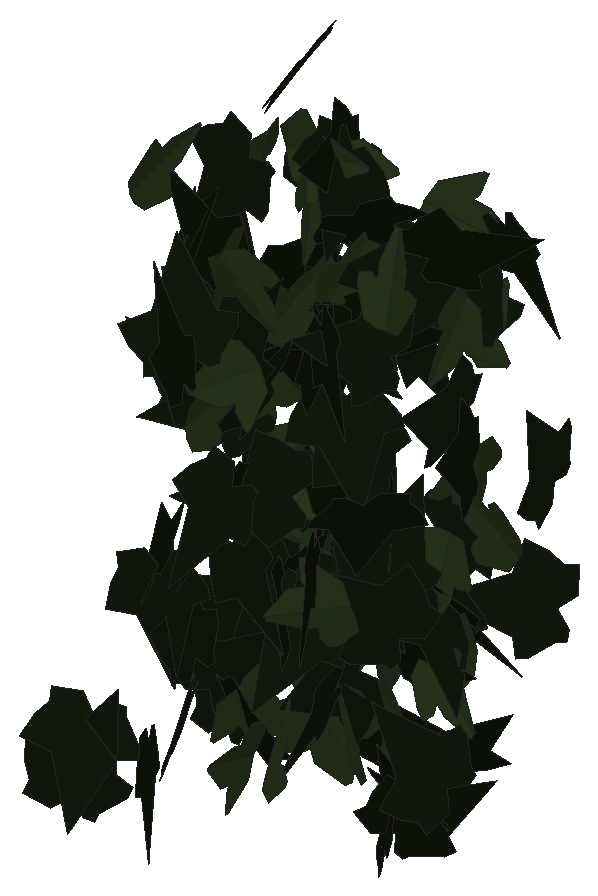
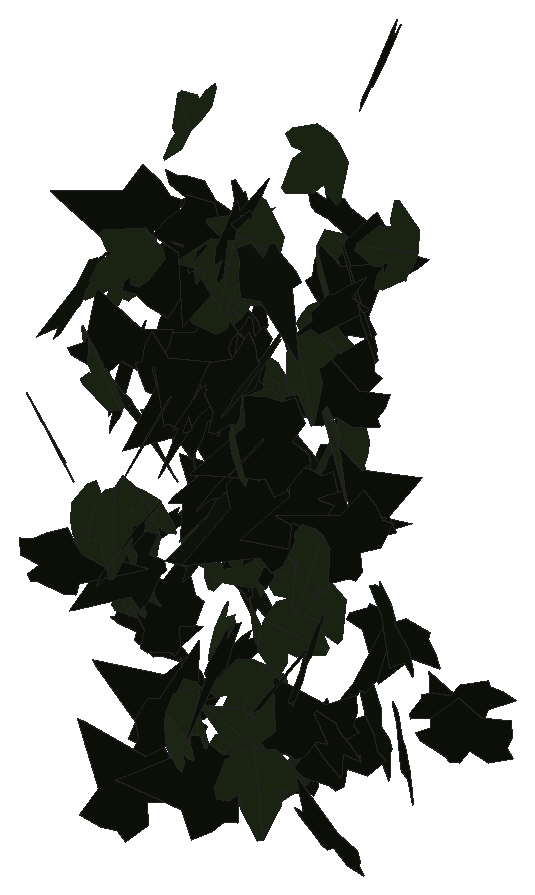
# SketchUp Ruby script. Lengths in inches.
U = 1.inch
M = Sketchup.active_model
def pt(a) = Geom::Point3d.new(a.map { |v| v * U })
def face(e, loops, mat)
  f = e.add_face(loops[0].map { |a| pt(a) })
  loops[1..].each { |l| e.add_face(l.map { |a| pt(a) }).erase! }
  f.material = f.back_material = mat if mat
  f
end
# faces: each face lists its corners as indices into pts; further lists are holes
def faces(e, pts, list, mat = nil) = list.each { |f| face(e, (f[0].is_a?(Array) ? f : [f]).map { |l| l.map { |i| pts[i] } }, mat) }
# xy, xz, yz: faces in a plane at the given z, y or x. An outline is a flat list of corners, or four numbers for a rectangle; further outlines are holes
def ring(l) = l.size == 4 ? [[l[0], l[1]], [l[2], l[1]], [l[2], l[3]], [l[0], l[3]]] : l.each_slice(2).to_a
def flat(e, list, mat, &to3) = list.each { |f| face(e, (f[0].is_a?(Array) ? f : [f]).map { |l| ring(l).map { |u, v| to3.(u, v) } }, mat) }
def xy(e, z, list, mat = nil) = flat(e, list, mat) { |x, y| [x, y, z] }
def xz(e, y, list, mat = nil) = flat(e, list, mat) { |x, z| [x, y, z] }
def yz(e, x, list, mat = nil) = flat(e, list, mat) { |y, z| [x, y, z] }
def lines(e, pts, list) = list.each { |a, b| e.add_line(pt(pts[a]), pt(pts[b])) }
# prism: a flat outline (further loops are holes) pulled along v
def prism(e, loops, v, mat = nil)
  f = face(e, loops, mat); d = Geom::Vector3d.new(v.map { |x| x * U })
  f.pushpull(f.normal.samedirection?(d) ? d.length : -d.length)
end
def box(e, o, s, mat = nil) = prism(e, [[o, [o[0] + s[0], o[1], o[2]], [o[0] + s[0], o[1] + s[1], o[2]], [o[0], o[1] + s[1], o[2]]]], [0, 0, s[2]], mat)
def at(x, y, z, deg = 0) = Geom::Transformation.translation(pt([x, y, z])) * Geom::Transformation.rotation(ORIGIN, Z_AXIS, deg.degrees)
def axes(o, x, y, z) = Geom::Transformation.new([*x, 0, *y, 0, *z, 0, *pt(o).to_a, 1])
def part(name) = M.definitions.add(name)
# library, detail: a bought-in or finely detailed component or shape, given as its bounding box
def library(name, o, s) = part(name).tap { |d| box(d.entities, o, s) }
def detail(e, o, s) = box(e.add_group.entities, o, s)
def put(e, d, t, mat = nil) = e.add_instance(d, t).tap { |i| i.material = mat if mat }
def group(e, t, mat = nil) = e.add_group.tap { |g| g.transformation = t; g.material = mat if mat }.entities
root = M.entities
M.materials.add("efeu1").color = [18, 25, 13]
M.materials.add("efeu2").color = [43, 57, 29]
c1 = part("ivyleaf_10")
p = [[0,0.5,-0.03],[-0.0625,2.02,-0.43],[-0.19,2.01,-0.46],[-0.54,1.05,-0.29],[-0.52,0.625,-0.18],[-0.83,0.76,-0.28],
  [-1.16,0.64,-0.33],[-1.15,0.33,-0.24],[-0.77,-0.39,0.02],[-0.3,-0.51,0.16],[0.04,-0.48,0.23],[-0.02,2.01,-0.4375],
  [-0.06,2.01,-0.43],[0.04,-0.49,0.23],[0.67,-0.49,0.14],[1.38,0.36,-0.2],[1.375,0.51,-0.24],[0.81,0.65,-0.19],
  [0.62,0.59,-0.15],[0.6,1.09,-0.28],[0.5,1.23,-0.31]]
faces(c1.entities,p,[[0,1,2,3,4,5,6,7,8,9,10],[11,12,0,13,14,15,16,17,18,19,20]],"efeu2")
c2 = part("ivyleaf_9")
p = [[1.54,2.16,1.25],[1.36,2.04,1.19],[-0.21,0.99,0.68],[-0.71,1.11,0.82],[-0.85,0.86,0.67],[-0.8,0.17,0.21],
  [-0.9,-0.01,0.1],[-0.67,-0.16,-0.02],[-0.08,-0.08,-0.05],[-0.03,-0.6,-0.4],[0.65,-0.88,-0.66],[0.83,-0.6,-0.49],
  [1.29,-0.42,-0.43],[1.8125,-0.07,-0.26],[1.21,0.44,0.15]]
faces(c2.entities,p,[[0,1,2,3,4,5,6,7,8,9,10,11,12,13,14]],"efeu1")
put(root,c1,axes([39.3,222.3,218.73],[-0.44801,0.21551,-0.05329],[0.04622,-0.02685,-0.49713],[-0.21713,-0.45037,0.00414]))
put(root,c2,axes([39.62,220.08,216.47],[-0.0302,0.25565,0.42864],[-0.09039,0.41952,-0.25658],[-0.49083,-0.09298,0.02087]))
put(root,c2,axes([39.49,221.64,213.66],[-0.36439,0.2665,0.21494],[0.16582,-0.13726,0.45129],[0.29954,0.40017,0.01165]))
put(root,c2,axes([39.87,220.75,218.66],[0.00532,0.02765,0.49921],[-0.44859,0.22071,-0.00744],[-0.22077,-0.4478,0.02716]))
put(root,c2,axes([39.52,218.93,214.83],[-0.25585,-0.4171,-0.10278],[0.05191,0.08873,-0.48932],[0.42643,-0.26106,-0.0021]))
put(root,c2,axes([39.48,218.61,213.9],[-0.34655,0.01099,0.36026],[0.35709,-0.05735,0.34525],[0.04891,0.49658,0.0319]))
put(root,c2,axes([39.36,221.26,218.25],[-0.01472,-0.00947,0.49969],[0.43968,0.23744,0.01745],[-0.23762,0.43992,0.00133]))
put(root,c2,axes([39.3125,222.43,217],[0.20074,-0.12423,-0.44076],[0.38837,-0.20881,0.23573],[-0.24265,-0.43699,0.01266]))
put(root,c1,axes([39.67,222.1,221.64],[0.0543,-0.49697,-0.00844],[0.00005,0.0085,-0.49993],[0.49704,0.05429,0.00097]))
put(root,c1,axes([39.84,221.24,220.02],[0.29275,-0.37958,-0.14219],[-0.0842,0.11462,-0.47934],[0.39649,0.3046,0.00319]))
put(root,c2,axes([40.08,221.4375,218.42],[-0.2695,-0.1346,0.39906],[-0.36868,-0.15361,-0.30079],[0.20357,-0.45639,-0.01645]))
put(root,c2,axes([39.66,220.1,216.45],[-0.28436,-0.21441,-0.35096],[0.28393,0.20633,-0.3561],[0.29753,-0.40181,0.00441]))
put(root,c1,axes([39.79,219.7,222.21],[0.08797,-0.2433,0.42786],[-0.05521,0.42702,0.25418],[-0.48909,-0.09197,0.04826]))
put(root,c1,axes([39.93,222.3,217.27],[-0.07929,-0.27273,0.4115],[-0.01679,-0.41504,-0.27831],[0.49339,-0.05795,0.05666]))
put(root,c2,axes([39.73,221.55,218.81],[0.16954,0.19203,0.42939],[0.26115,0.3412,-0.2557],[-0.39122,0.31098,0.0154]))
put(root,c2,axes([39.91,221.53,215.5],[-0.41786,-0.09545,-0.25745],[0.25174,0.05399,-0.42862],[0.10962,-0.48783,0.00293]))
put(root,c2,axes([40.07,220.25,215.38],[-0.12429,-0.3751,0.30635],[0.08668,0.29395,0.39507],[-0.47648,0.15132,-0.00804]))
put(root,c2,axes([39.74,222.57,216.5625],[0.14211,-0.47646,0.05281],[0.01344,-0.0511,-0.4972],[0.47919,0.14273,-0.00172]))
put(root,c2,axes([39.97,221.43,221.81],[-0.14993,-0.39085,0.27341],[-0.1041,-0.25288,-0.41859],[0.46549,-0.18244,-0.00554]))
put(root,c2,axes([39.9375,221.49,215.15],[-0.27909,-0.10822,0.4005],[0.37157,0.14948,0.29932],[-0.18452,0.4647,-0.00302]))
put(root,c2,axes([40.23,222.23,222.99],[-0.21232,0.44741,-0.06886],[0.02994,-0.06201,-0.49524],[-0.45169,-0.21442,-0.00046]))
put(root,c2,axes([40.08,220.82,220],[-0.41487,-0.07019,0.2701],[0.27115,0.01306,0.41989],[-0.066,0.49488,0.02723]))
put(root,c1,axes([40.17,221.32,218.69],[-0.35539,-0.35047,-0.02948],[0.02232,0.01935,-0.49913],[0.351,-0.35609,0.00189]))
put(root,c2,axes([40.27,219.6,214.38],[0.0029,0.19478,0.46049],[-0.01837,0.46023,-0.19455],[-0.49965,-0.01579,0.00983]))
put(root,c2,axes([39.84,220.9375,214.51],[-0.12861,0.01441,0.48296],[0.46818,-0.11982,0.12825],[0.11943,0.48522,0.01733]))
put(root,c2,axes([39.93,219.54,214.26],[-0.1694,0.00721,-0.47038],[0.46317,-0.08493,-0.1681],[-0.08232,-0.49268,0.02209]))
put(root,c2,axes([39.96,220.1875,220.98],[-0.07585,0.32165,0.37522],[0.08774,-0.36482,0.33047],[0.48636,0.11598,-0.0011]))
put(root,c1,axes([40.1,221.24,217.28],[-0.36769,-0.11561,-0.31849],[0.30097,0.10443,-0.38537],[0.15563,-0.47511,-0.0072]))
put(root,c1,axes([40.41,222.23,214.8125],[-0.41323,-0.27054,0.07777],[-0.06222,-0.04694,-0.49389],[0.27454,-0.41785,0.00513]))
put(root,c2,axes([40.0625,221.9375,220.04],[0.29327,0.19818,0.35315],[0.29639,0.19208,-0.35392],[-0.27595,0.41693,-0.00481]))
put(root,c2,axes([40.24,221.3,219.01],[0.33732,0.35149,0.11258],[0.07116,0.08772,-0.48708],[-0.36215,0.34462,0.00916]))
put(root,c2,axes([40.08,222.17,218.9375],[0.43106,0.14291,0.20921],[0.19332,0.08134,-0.45388],[-0.16376,0.47219,0.01487]))
put(root,c1,axes([40.43,219.97,218.95],[0.07725,-0.04196,0.49221],[-0.15093,0.47237,0.06396],[-0.47037,-0.15846,0.06032]))
put(root,c2,axes([40.67,220.06,221.18],[0.12898,-0.07058,0.47789],[-0.36175,0.31371,0.14396],[-0.32016,-0.38289,0.02986]))
put(root,c2,axes([40.17,222.55,221.35],[0.17411,-0.45097,0.12772],[0.04085,-0.12113,-0.48338],[0.46692,0.17875,-0.00534]))
put(root,c1,axes([40.49,220.76,214.69],[-0.14852,-0.36538,-0.30731],[0.13502,0.27656,-0.39406],[0.45794,-0.20004,0.01652]))
put(root,c2,axes([40.82,220.82,219.2],[-0.3644,0.34211,-0.01318],[0.00909,-0.00958,-0.49983],[-0.34224,-0.36452,0.00076]))
put(root,c1,axes([40.55,222.375,220.14],[0.17648,-0.40184,0.23955],[0.08987,-0.22214,-0.43884],[0.45911,0.19794,-0.00618]))
put(root,c2,axes([40.95,221.02,217.57],[-0.25824,-0.07879,0.42084],[-0.39445,-0.14735,-0.26963],[0.16651,-0.47125,0.01395]))
put(root,c2,axes([40.5,222.59,219.71],[0.10549,-0.48701,0.04114],[0.0131,-0.03925,-0.49828],[0.48857,0.1062,0.00448]))
put(root,c1,axes([40.67,221.24,219.85],[0.01529,-0.32853,0.37661],[-0.0147,0.37632,0.32888],[-0.49955,-0.02113,0.00185]))
put(root,c2,axes([40.41,220.83,214.29],[0.14982,-0.18464,0.43985],[0.27098,-0.34648,-0.23774],[0.39258,0.30962,-0.00375]))
put(root,c2,axes([40.73,219.92,219.69],[-0.12789,-0.13533,0.46404],[0.41546,0.21457,0.17707],[-0.24706,0.43087,0.05757]))
put(root,c2,axes([40.61,222.33,220.78],[0.22982,-0.28587,0.3398],[0.22344,-0.2562,-0.36666],[0.38374,0.32038,0.00999]))
put(root,c2,axes([40.97,222.2,216.6],[0.23182,-0.19665,-0.39697],[-0.3012,0.25858,-0.30399],[0.32486,0.38008,0.00142]))
put(root,c1,axes([40.89,221.42,217.42],[0.42368,0.16613,-0.20712],[0.13566,0.19983,0.43779],[0.22824,-0.42716,0.12425]))
put(root,c1,axes([40.78,221.6,214.71],[-0.23927,-0.13519,0.4177],[0.36256,0.20744,0.27481],[-0.2476,0.43439,-0.00124]))
put(root,c1,axes([41.05,219.85,221.7],[0.20607,-0.42795,0.15619],[0.07588,-0.13679,-0.4749],[0.4492,0.21943,0.00856]))
put(root,c2,axes([41.1875,219.48,218.49],[-0.17767,0.21448,-0.41525],[0.27559,-0.31071,-0.2784],[-0.37747,-0.3278,-0.00781]))
put(root,c2,axes([41.38,218.5,220.91],[-0.46383,-0.1176,0.14502],[0.14023,0.03697,0.47851],[-0.12327,0.48457,-0.00131]))
put(root,c1,axes([41.03,221.45,216.75],[0.32857,-0.20091,0.31887],[0.27158,-0.1671,-0.38513],[0.26131,0.42628,-0.00068]))
put(root,c1,axes([41.57,219.36,220.27],[0.29202,-0.0677,-0.40017],[-0.38726,0.10107,-0.2997],[0.12147,0.48498,0.0066]))
put(root,c1,axes([41.26,221.2,222.07],[-0.02616,0.43415,-0.24663],[0.00712,-0.24662,-0.43489],[-0.49926,-0.02626,0.00672]))
put(root,c1,axes([41.43,221.29,214.36],[-0.33069,-0.36139,-0.1002],[0.068,0.0736,-0.48986],[0.36881,-0.33761,0.00047]))
put(root,c1,axes([41.07,221.15,222.43],[-0.08189,-0.04115,0.49153],[0.4757,0.12512,0.08973],[-0.13038,0.48234,0.01866]))
put(root,c2,axes([41.18,221.34,217.28],[-0.05181,0.06609,0.4929],[0.30622,-0.38623,0.08398],[0.39185,0.31057,-0.00046]))
put(root,c2,axes([41.45,222.0625,220.375],[0.24263,-0.31489,-0.30327],[-0.18063,0.24365,-0.3975],[0.39812,0.30245,0.00448]))
put(root,c2,axes([41.54,221.49,222.3125],[-0.01556,-0.08629,0.49225],[-0.14127,-0.47164,-0.08715],[0.47938,-0.14179,-0.00971]))
put(root,c1,axes([41.52,221.37,222.33],[0.31445,0.38338,0.06432],[0.04083,0.0497,-0.49585],[-0.38659,0.31709,-0.00005]))
put(root,c2,axes([41.33,221.94,214.16],[0.15993,0.15414,-0.44796],[0.28679,0.34481,0.22103],[0.37706,-0.32764,0.02188]))
put(root,c1,axes([41.6875,220.61,215.0625],[-0.35445,-0.27769,-0.21739],[0.16749,0.13868,-0.45024],[0.31034,-0.39199,-0.00529]))
put(root,c2,axes([41.66,221.41,222.51],[-0.08244,-0.48339,0.09766],[-0.02195,-0.09533,-0.49034],[0.49267,-0.08514,-0.0055]))
put(root,c2,axes([41.51,221.81,218.01],[0.31439,-0.38067,0.07904],[0.05027,-0.061,-0.49371],[0.38553,0.31838,-0.00009]))
put(root,c1,axes([41.78,222.27,215.09],[0.14468,-0.38115,0.28947],[0.09589,-0.27319,-0.40764],[0.46891,0.17347,-0.00595]))
put(root,c2,axes([41.92,220.4,220.33],[0.05014,-0.05989,-0.49386],[-0.35717,0.34118,-0.07763],[0.34629,0.36057,-0.00856]))
put(root,c2,axes([42.12,222.1875,220.19],[0.07208,-0.09724,0.48513],[-0.32056,0.36426,0.12065],[-0.37689,-0.32842,-0.00983]))
put(root,c2,axes([41.95,219.76,217.26],[-0.06999,0.13346,-0.47675],[-0.19823,0.43365,0.1505],[0.45366,0.21008,-0.00779]))
put(root,c1,axes([41.99,220.33,217.33],[0.1091,-0.4869,-0.03201],[-0.00697,0.03125,-0.49897],[0.4879,0.10932,0.00003]))
put(root,c2,axes([41.78,221.34,218.62],[0.05428,-0.42395,-0.25947],[-0.00199,0.26082,-0.42658],[0.49704,0.04734,0.02662]))
put(root,c2,axes([41.95,221.13,215.35],[0.13326,-0.29625,-0.3801],[0.1467,-0.35071,0.32478],[-0.45904,-0.19808,-0.00655]))
put(root,c1,axes([42.31,221.41,214.74],[0.02369,-0.01707,-0.49915],[-0.34222,0.36341,-0.02867],[0.36377,0.34299,0.00554]))
put(root,c2,axes([42.08,221.64,219.99],[-0.09063,0.17684,-0.45882],[-0.19573,0.41502,0.19862],[0.45108,0.21561,-0.006]))
put(root,c2,axes([41.65,220.87,220.19],[0.1538,-0.04409,-0.47371],[0.44104,0.19991,0.12458],[0.17842,-0.45617,0.10038]))
put(root,c2,axes([41.96,220.94,219.3],[-0.15577,-0.41624,-0.22908],[0.10804,0.20373,-0.44365],[0.46267,-0.18771,0.02647]))
put(root,c1,axes([42.03,220.78,221.04],[-0.04763,-0.45093,0.21069],[0.02318,0.20941,0.45344],[-0.49719,0.05296,0.00095]))
put(root,c1,axes([42.03,219.93,216.53],[0.29242,0.33978,-0.22144],[0.12995,0.18011,0.44796],[0.38419,-0.31954,0.01703]))
put(root,c2,axes([42.15,221.93,220.02],[0.30808,-0.29687,-0.25875],[-0.1782,0.18787,-0.42772],[0.35118,0.35577,0.00995]))
put(root,c2,axes([42.29,220.7,222.14],[0.28606,0.40883,-0.03206],[-0.0204,-0.02485,-0.49897],[-0.40958,0.28677,0.00247]))
put(root,c2,axes([41.92,221.09,220.17],[0.20062,-0.04302,0.45596],[0.45416,-0.04553,-0.20413],[0.05909,0.49606,0.02081]))
put(root,c1,axes([42,221.16,217.24],[0.09299,-0.11253,0.47821],[0.47523,-0.10276,-0.11659],[0.12453,0.47621,0.08785]))
put(root,c1,axes([42.2,218.42,222.375],[-0.39768,0.09056,-0.28923],[0.28393,-0.05558,-0.40779],[-0.10601,-0.48858,-0.00721]))
put(root,c2,axes([42.13,219.53,217.3],[0.13525,-0.09251,-0.47239],[0.42468,-0.20808,0.16234],[-0.22662,-0.44514,0.02229]))
put(root,c2,axes([42.33,220.3,217.45],[-0.00424,-0.28361,-0.41176],[0.08206,0.4058,-0.28035],[0.4932,-0.06995,0.0431]))
put(root,c2,axes([42.27,222.38,213.74],[0.38943,0.30413,-0.07651],[0.06025,0.04715,0.49411],[0.30776,-0.39406,0.00008]))
put(root,c2,axes([42.68,219.39,217.24],[-0.41022,-0.28537,-0.017],[0.01689,0.0055,-0.49968],[0.28537,-0.41053,0.00513]))
put(root,c1,axes([42.86,220.01,214.91],[-0.25583,0.298,-0.30943],[-0.2031,0.23345,0.39275],[0.37855,0.32664,0.0016]))
put(root,c2,axes([42.83,219.56,216.07],[-0.38792,0.20739,-0.23771],[0.19593,-0.13689,-0.43917],[-0.24724,-0.43388,0.02494]))
put(root,c2,axes([43.09,221.24,221.45],[-0.12697,-0.12506,-0.46716],[-0.27881,-0.37572,0.17636],[-0.39515,0.30528,0.02567]))
put(root,c2,axes([42.56,217.97,218.72],[0.2473,-0.39665,-0.17752],[-0.08825,0.15416,-0.46738],[0.4255,0.2625,0.00624]))
put(root,c1,axes([42.88,222.26,218.16],[-0.08173,-0.48524,-0.08866],[0.02918,0.08495,-0.49187],[0.49241,-0.08557,0.01443]))
put(root,c1,axes([42.82,217.89,215.86],[-0.04996,-0.15787,-0.47179],[-0.03187,-0.47217,0.16137],[-0.49648,0.04619,0.03712]))
put(root,c2,axes([42.76,219.66,216.99],[-0.16303,-0.09729,0.46256],[0.42096,0.19264,0.18888],[-0.21497,0.45103,0.0191]))
put(root,c2,axes([43.3,221.44,219.34],[-0.30657,0.33204,0.21393],[-0.13759,0.16407,-0.45183],[-0.37025,-0.3359,-0.00923]))
put(root,c2,axes([42.98,220.98,213.82],[0.40686,-0.24652,0.15392],[-0.13023,0.08208,0.47571],[-0.25981,-0.42719,0.00258]))
put(root,c2,axes([43.2,220.15,213.79],[0.00324,0.05013,0.49747],[-0.0734,0.49214,-0.04911],[-0.49457,-0.07271,0.01055]))
put(root,c2,axes([42.87,222.16,217.39],[-0.00839,-0.41309,0.28158],[-0.01014,-0.28142,-0.41316],[0.49983,-0.01265,-0.00365]))
put(root,c2,axes([43.16,216.15,222.18],[-0.03414,-0.36425,0.34082],[0.03003,0.3395,0.36584],[-0.49793,0.04545,-0.0013]))
put(root,c2,axes([43.03,221.9375,220.35],[-0.36778,-0.10519,0.32198],[0.31973,0.04911,0.38126],[-0.11183,0.48634,0.03115]))
put(root,c1,axes([42.875,221.6875,221.99],[0.09586,0.26838,0.41083],[0.13793,0.38698,-0.28499],[-0.47094,0.16797,0.00016]))
put(root,c2,axes([42.7,221.13,215.86],[0.1483,-0.12018,0.46213],[0.36603,-0.28214,-0.19083],[0.30664,0.39491,0.0043]))
put(root,c1,axes([42.91,222.35,220],[0.38893,-0.20551,-0.23769],[0.20985,-0.11163,0.43989],[-0.23387,-0.44193,-0.00058]))
put(root,c2,axes([43.45,219.93,218.49],[-0.01857,-0.00101,-0.49965],[-0.4824,0.1303,0.01766],[0.13018,0.48272,-0.00581]))
put(root,c2,axes([42.9375,219.23,221.37],[-0.09035,-0.02406,-0.49118],[0.49169,-0.01333,-0.08979],[-0.00877,-0.49924,0.02607]))
put(root,c1,axes([43.64,221.94,217.4375],[-0.25835,0.09063,-0.41838],[-0.39853,0.12751,0.27371],[0.15631,0.4749,0.00636]))
put(root,c2,axes([43.44,216.76,220.4],[-0.48223,-0.0677,-0.11345],[0.11221,0.01678,-0.48696],[0.06974,-0.49511,-0.00099]))
put(root,c1,axes([43.7,221.11,216.37],[0.09211,-0.09285,-0.48259],[-0.34654,0.33588,-0.13076],[0.34847,0.35856,-0.00247]))
put(root,c1,axes([43.36,221.08,217.59],[0.48804,-0.10562,0.02572],[0.02562,-0.00319,-0.49933],[0.10565,0.48871,0.0023]))
put(root,c2,axes([43.18,221.2,216.8125],[0.49333,-0.06311,0.05138],[0.05108,-0.00558,-0.49735],[0.06335,0.49597,0.00094]))
put(root,c2,axes([43.22,220.41,213.87],[0.00895,-0.04662,0.49774],[0.49893,0.0322,-0.00596],[-0.0315,0.49678,0.04709]))
put(root,c2,axes([43.95,219.25,221.39],[-0.33245,0.13964,0.34637],[-0.32486,0.12064,-0.36044],[-0.18424,-0.4647,0.01051]))
put(root,c2,axes([43.4,220.98,216.95],[0.04606,-0.48878,-0.0947],[-0.00884,0.09429,-0.49095],[0.4978,0.0469,0.00004]))
put(root,c2,axes([43.32,222.4375,221.53],[0.32348,-0.38054,-0.02339],[-0.0164,0.01676,-0.49945],[0.38091,0.32389,-0.00164]))
put(root,c1,axes([44,218.14,218.33],[-0.16148,-0.05636,0.46984],[-0.42357,-0.20412,-0.17006],[0.21098,-0.45294,0.01818]))
put(root,c2,axes([44.04,220.26,214.875],[-0.42559,-0.14105,-0.2213],[-0.20835,-0.07475,0.44833],[-0.15956,0.47383,0.00485]))
put(root,c1,axes([43.32,220.95,215.97],[0.24827,-0.00908,0.43391],[0.43365,-0.01512,-0.24843],[0.01763,0.49969,0.00036]))
put(root,c2,axes([43.66,219.53,217.97],[-0.36764,0.00764,0.33879],[0.33654,-0.05035,0.36634],[0.03971,0.4974,0.03188]))
put(root,c1,axes([43.69,221.07,221.08],[0.01424,0.30388,-0.39681],[-0.03519,-0.39537,-0.30404],[-0.49856,0.03659,0.01012]))
put(root,c2,axes([43.36,220.91,221.85],[0.15194,-0.01798,0.47602],[0.47635,0.00419,-0.15189],[0.00147,0.49966,0.0184]))
put(root,c2,axes([43.96,218.78,219.4375],[0.18677,0.40634,-0.22363],[-0.08875,-0.20531,-0.44718],[-0.45524,0.20673,-0.00457]))
put(root,c2,axes([43.79,221.125,218.98],[-0.00196,-0.05348,0.49713],[-0.0817,-0.49042,-0.05308],[0.49328,-0.08143,-0.00681]))
put(root,c1,axes([43.81,217.14,216.36],[0.34929,-0.35748,-0.01434],[0.01058,-0.00971,0.49979],[-0.35761,-0.34945,0.00078]))
put(root,c2,axes([44.29,222.09,216.68],[-0.27477,-0.02939,0.4167],[-0.41515,-0.03615,-0.2763],[0.04637,-0.49782,-0.00454]))
put(root,c2,axes([43.88,217.875,219.11],[-0.0829,0.03755,-0.49165],[0.44258,-0.21412,-0.09098],[-0.21738,-0.45027,0.00226]))
put(root,c2,axes([44.48,218.76,217.83],[-0.02066,0.07228,0.49432],[-0.49954,0.00293,-0.02131],[-0.00597,-0.49474,0.07209]))
put(root,c2,axes([44.53,221.8125,218.72],[-0.31943,0.09266,-0.37333],[-0.36587,0.07663,0.33206],[0.11876,0.48533,0.01885]))
put(root,c1,axes([44.24,218.86,222.32],[0.03053,0.40329,-0.29398],[-0.00734,0.29486,0.40374],[0.49901,-0.02034,0.02393]))
